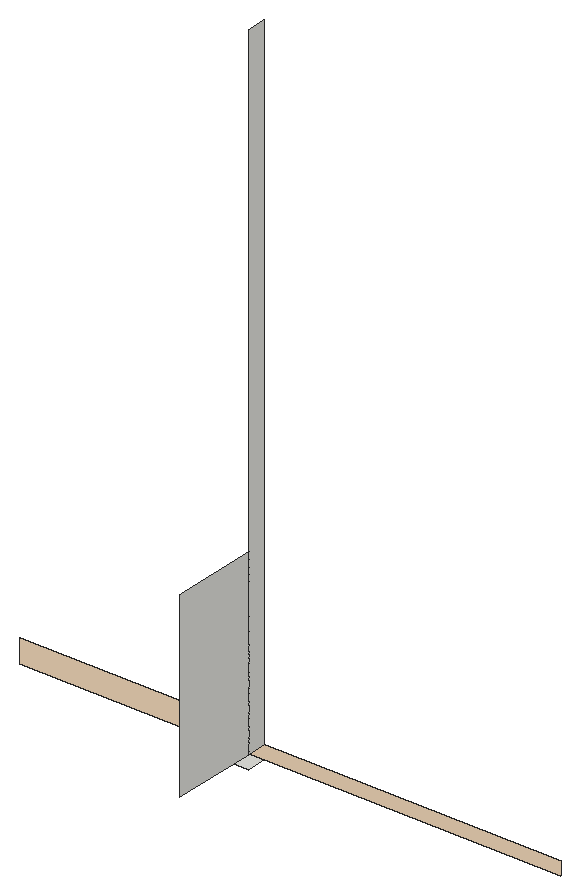
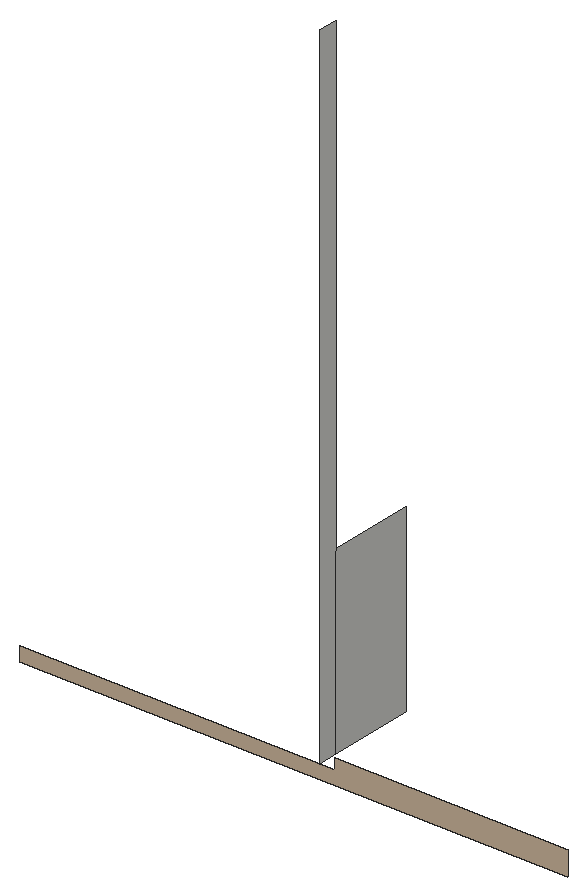
# SketchUp Ruby script. Lengths in inches.
U = 1.inch
M = Sketchup.active_model
def pt(a) = Geom::Point3d.new(a.map { |v| v * U })
def face(e, loops, mat)
  f = e.add_face(loops[0].map { |a| pt(a) })
  loops[1..].each { |l| e.add_face(l.map { |a| pt(a) }).erase! }
  f.material = f.back_material = mat if mat
  f
end
# faces: each face lists its corners as indices into pts; further lists are holes
def faces(e, pts, list, mat = nil) = list.each { |f| face(e, (f[0].is_a?(Array) ? f : [f]).map { |l| l.map { |i| pts[i] } }, mat) }
# xy, xz, yz: faces in a plane at the given z, y or x. An outline is a flat list of corners, or four numbers for a rectangle; further outlines are holes
def ring(l) = l.size == 4 ? [[l[0], l[1]], [l[2], l[1]], [l[2], l[3]], [l[0], l[3]]] : l.each_slice(2).to_a
def flat(e, list, mat, &to3) = list.each { |f| face(e, (f[0].is_a?(Array) ? f : [f]).map { |l| ring(l).map { |u, v| to3.(u, v) } }, mat) }
def xy(e, z, list, mat = nil) = flat(e, list, mat) { |x, y| [x, y, z] }
def xz(e, y, list, mat = nil) = flat(e, list, mat) { |x, z| [x, y, z] }
def yz(e, x, list, mat = nil) = flat(e, list, mat) { |y, z| [x, y, z] }
def lines(e, pts, list) = list.each { |a, b| e.add_line(pt(pts[a]), pt(pts[b])) }
# prism: a flat outline (further loops are holes) pulled along v
def prism(e, loops, v, mat = nil)
  f = face(e, loops, mat); d = Geom::Vector3d.new(v.map { |x| x * U })
  f.pushpull(f.normal.samedirection?(d) ? d.length : -d.length)
end
def box(e, o, s, mat = nil) = prism(e, [[o, [o[0] + s[0], o[1], o[2]], [o[0] + s[0], o[1] + s[1], o[2]], [o[0], o[1] + s[1], o[2]]]], [0, 0, s[2]], mat)
def at(x, y, z, deg = 0) = Geom::Transformation.translation(pt([x, y, z])) * Geom::Transformation.rotation(ORIGIN, Z_AXIS, deg.degrees)
def axes(o, x, y, z) = Geom::Transformation.new([*x, 0, *y, 0, *z, 0, *pt(o).to_a, 1])
def part(name) = M.definitions.add(name)
# library, detail: a bought-in or finely detailed component or shape, given as its bounding box
def library(name, o, s) = part(name).tap { |d| box(d.entities, o, s) }
def detail(e, o, s) = box(e.add_group.entities, o, s)
def put(e, d, t, mat = nil) = e.add_instance(d, t).tap { |i| i.material = mat if mat }
def group(e, t, mat = nil) = e.add_group.tap { |g| g.transformation = t; g.material = mat if mat }.entities
root = M.entities
M.materials.add("[0012_Bisque]3").color = [255, 228, 196]
xy(root,95.625,[[202.72,476.15,211.5,487.49]])
xz(root,487.49,[[65.97,95.625,65.97,109.8125,202.72,109.8125,202.72,103.6875,388.14,103.6875,388.14,95.625]],"[0012_Bisque]3")
yz(root,211.5,[[424.53,103.6875,475.86,211.6875],[475.86,103.6875,487.49,490.375]])
